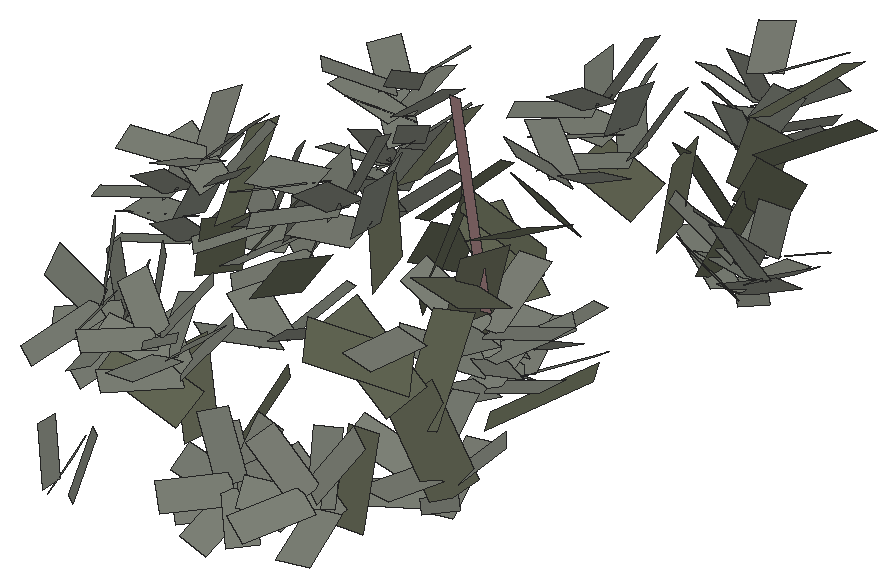
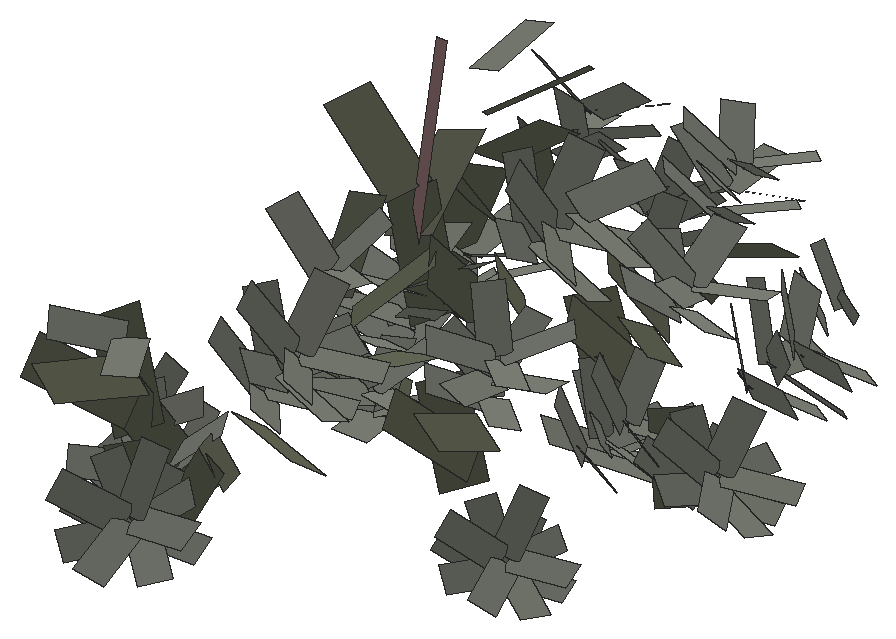
# SketchUp Ruby script. Lengths in inches.
U = 1.inch
M = Sketchup.active_model
def pt(a) = Geom::Point3d.new(a.map { |v| v * U })
def face(e, loops, mat)
  f = e.add_face(loops[0].map { |a| pt(a) })
  loops[1..].each { |l| e.add_face(l.map { |a| pt(a) }).erase! }
  f.material = f.back_material = mat if mat
  f
end
# faces: each face lists its corners as indices into pts; further lists are holes
def faces(e, pts, list, mat = nil) = list.each { |f| face(e, (f[0].is_a?(Array) ? f : [f]).map { |l| l.map { |i| pts[i] } }, mat) }
# xy, xz, yz: faces in a plane at the given z, y or x. An outline is a flat list of corners, or four numbers for a rectangle; further outlines are holes
def ring(l) = l.size == 4 ? [[l[0], l[1]], [l[2], l[1]], [l[2], l[3]], [l[0], l[3]]] : l.each_slice(2).to_a
def flat(e, list, mat, &to3) = list.each { |f| face(e, (f[0].is_a?(Array) ? f : [f]).map { |l| ring(l).map { |u, v| to3.(u, v) } }, mat) }
def xy(e, z, list, mat = nil) = flat(e, list, mat) { |x, y| [x, y, z] }
def xz(e, y, list, mat = nil) = flat(e, list, mat) { |x, z| [x, y, z] }
def yz(e, x, list, mat = nil) = flat(e, list, mat) { |y, z| [x, y, z] }
def lines(e, pts, list) = list.each { |a, b| e.add_line(pt(pts[a]), pt(pts[b])) }
# prism: a flat outline (further loops are holes) pulled along v
def prism(e, loops, v, mat = nil)
  f = face(e, loops, mat); d = Geom::Vector3d.new(v.map { |x| x * U })
  f.pushpull(f.normal.samedirection?(d) ? d.length : -d.length)
end
def box(e, o, s, mat = nil) = prism(e, [[o, [o[0] + s[0], o[1], o[2]], [o[0] + s[0], o[1] + s[1], o[2]], [o[0], o[1] + s[1], o[2]]]], [0, 0, s[2]], mat)
def at(x, y, z, deg = 0) = Geom::Transformation.translation(pt([x, y, z])) * Geom::Transformation.rotation(ORIGIN, Z_AXIS, deg.degrees)
def axes(o, x, y, z) = Geom::Transformation.new([*x, 0, *y, 0, *z, 0, *pt(o).to_a, 1])
def part(name) = M.definitions.add(name)
# library, detail: a bought-in or finely detailed component or shape, given as its bounding box
def library(name, o, s) = part(name).tap { |d| box(d.entities, o, s) }
def detail(e, o, s) = box(e.add_group.entities, o, s)
def put(e, d, t, mat = nil) = e.add_instance(d, t).tap { |i| i.material = mat if mat }
def group(e, t, mat = nil) = e.add_group.tap { |g| g.transformation = t; g.material = mat if mat }.entities
root = M.entities
M.materials.add("tak1dsfasd0f156w").color = [150, 118, 119]
M.materials.add("viburnumblaasdfas0df1w06d").color = [98, 102, 84]
M.materials.add("viburnumbladsadfasdfad0w122").color = [125, 129, 119]
c1 = part("Component\#315")
p = [[0.25,0,0],[2.05,0.01,0.35],[1.81,4.2,1.66],[0,4.19,1.3125]]
faces(c1.entities,p,[[0,1,2,3]],"viburnumbladsadfasdfad0w122")
c2 = part("viburnumblad2")
put(c2.entities,c1,axes([-19.23,-4.49,-32.18],[83.35428,0,0],[0,79.38502,0],[0,0,83.35428]))
c3 = part("Component\#314")
p = [[0.14,0,0],[2.58,0.05,0.25],[2.44,5.11,2.64],[0,5.05,2.39]]
faces(c3.entities,p,[[0,1,2,3]],"viburnumblaasdfas0df1w06d")
c4 = part("viburnumblad1\#2")
put(c4.entities,c3,axes([-37.25,6.23,19.31],[75.98784,0,0],[0,65.50676,0],[0,0,75.98784]))
c5 = part("Component\#337")
p = [[0.6,0,12.07],[1.51,1.22,0.03],[0.91,1.23,0],[0,0,12.04]]
faces(c5.entities,p,[[0,1,2,3]],"tak1dsfasd0f156w")
put(root,c2,axes([1233.48,184.79,34.33],[-0.00995,0.00489,0.00397],[-0.00628,-0.00876,-0.0047],[0.00102,-0.00608,0.00892]))
put(root,c2,axes([1233.86,186.39,33.78],[-0.01153,-0.00217,-0.00126],[0.00257,-0.00998,-0.00587],[-0.00007,-0.00594,0.00905]))
put(root,c2,axes([1227.22,186.21,31.97],[-0.00593,0.00534,0.00783],[-0.0086,-0.00691,-0.00181],[0.00397,-0.00698,0.00778]))
put(root,c2,axes([1232.86,185.47,33.13],[-0.00254,0.00908,0.00688],[-0.01141,-0.00302,-0.00024],[0.00165,-0.00679,0.00837]))
put(root,c2,axes([1227.72,187.22,32.82],[-0.00902,-0.00601,-0.00274],[0.00624,-0.00625,-0.00686],[0.00215,-0.00706,0.0084]))
put(root,c2,axes([1231.99,184.72,34.32],[0.00636,0.00796,0.00575],[-0.00984,0.00398,0.00495],[0.00146,-0.00765,0.00773]))
put(root,c2,axes([1215.61,186.57,29.77],[0.00345,-0.00905,-0.004],[0.00788,-0.00012,0.00668],[-0.00594,-0.00519,0.00581]))
put(root,c2,axes([1227.25,187.8,31.45],[-0.01058,-0.00047,0.0036],[-0.00191,-0.00936,-0.00683],[0.00314,-0.00674,0.00835]))
put(root,c2,axes([1231.93,185.9,35.2],[0.00995,-0.00489,-0.00397],[0.00634,0.00703,0.00672],[-0.00053,-0.00802,0.00751]))
put(root,c2,axes([1214.98,185.86,28.87],[0.00855,0.00051,0.00592],[-0.00403,0.00835,0.00477],[-0.00448,-0.00623,0.00604]))
put(root,c2,axes([1226.24,187.05,31.04],[0.00218,0.00802,0.00747],[-0.00931,-0.0013,0.00412],[0.00416,-0.00766,0.007]))
put(root,c2,axes([1225.95,186.33,32.57],[0.00902,0.00601,0.00274],[-0.00554,0.00435,0.00868],[0.0036,-0.00837,0.00649]))
put(root,c2,axes([1226.29,188.11,30.18],[-0.0062,0.00558,0.00817],[-0.00774,-0.00622,-0.00163],[0.00397,-0.00698,0.00778]))
put(root,c2,axes([1215.79,186.9,28.39],[0.00848,-0.00604,0.00136],[0.00312,0.00638,0.00815],[-0.00533,-0.00595,0.00568]))
put(root,c2,axes([1231.8,186.11,33.61],[0.01153,0.00217,0.00126],[-0.00261,0.00855,0.00823],[0.00055,-0.00816,0.00738]))
put(root,c2,axes([1232.29,186.56,32.28],[0.00611,0.00764,0.00552],[-0.01063,0.0043,0.00535],[0.00146,-0.00765,0.00773]))
put(root,c2,axes([1226.45,187.34,33.43],[0.00593,-0.00534,-0.00783],[0.00931,0.00502,0.00364],[0.00177,-0.00845,0.00711]))
put(root,c2,axes([1226.68,188.44,32.37],[-0.00218,-0.00802,-0.00747],[0.01085,-0.00048,-0.00266],[0.00158,-0.00777,0.00788]))
put(root,c2,axes([1220.38,188.49,37.75],[-0.00773,0.00806,0.00054],[-0.00787,-0.00734,-0.00302],[-0.00183,-0.00247,0.01075]))
put(root,c2,axes([1221.09,189.64,36.78],[-0.01083,0.00076,-0.00267],[-0.00024,-0.01097,-0.00215],[-0.00276,-0.00202,0.01064]))
put(root,c2,axes([1220.6,189.8,38.24],[-0.00759,-0.00699,-0.00431],[0.00733,-0.00841,0.00072],[-0.00369,-0.00233,0.01029]))
put(root,c2,axes([1225.42,187.78,32.17],[0.01058,0.00047,-0.0036],[0.00255,0.00709,0.00842],[0.00261,-0.00869,0.00653]))
put(root,c2,axes([1221.08,189.65,35.28],[-0.00742,0.00774,0.00052],[-0.0085,-0.00793,-0.00326],[-0.00183,-0.00247,0.01075]))
put(root,c2,axes([1225.21,188.11,30.72],[0.0079,0.00633,0.00186],[-0.00554,0.00435,0.00868],[0.00455,-0.00767,0.00675]))
put(root,c2,axes([1220.16,188.9375,36.28],[-0.0001,0.01064,0.00343],[-0.01164,0.00037,-0.00146],[-0.00143,-0.00341,0.01055]))
put(root,c4,axes([1231.6875,189.11,30.82],[0.01273,-0.00184,0.00122],[0.00029,0.0105,0.01027],[-0.0024,-0.00896,0.00784]))
put(root,c2,axes([1220.25,190.8,36.92],[0.0001,-0.01064,-0.00343],[0.01052,-0.00118,0.00394],[-0.00407,-0.00322,0.0099]))
put(root,c2,axes([1219.03,188.81,37.5],[0.00759,0.00699,0.00431],[-0.00801,0.0076,0.00179],[-0.00181,-0.0043,0.01016]))
put(root,c2,axes([1219.25,190.12,37.98],[0.00773,-0.00806,-0.00054],[0.0072,0.00653,0.00553],[-0.00368,-0.00417,0.0097]))
put(root,c4,axes([1220.77,190.28,32.375],[0.0023,0.0101,0.00657],[-0.0138,0.00343,-0.00044],[-0.0019,-0.0063,0.01035]))
put(root,c2,axes([1219.1875,189.82,36.29],[0.01083,-0.00076,0.00267],[-0.0004,0.00932,0.00428],[-0.00274,-0.00461,0.00981]))
put(root,c2,axes([1233.8,193.38,40.56],[-0.01204,0.00026,0.00058],[-0.00039,-0.0134,-0.00212],[0.00055,-0.00198,0.01239]))
put(root,c2,axes([1219.7,189.85,35.01],[0.00793,0.00729,0.0045],[-0.00721,0.00684,0.00161],[-0.00181,-0.0043,0.01016]))
put(root,c2,axes([1219.8125,190.96,35.5],[0.00743,-0.00696,-0.00145],[0.0072,0.00653,0.00553],[-0.00282,-0.00502,0.00959]))
put(root,c4,axes([1233.05,193.24,37.29],[-0.00623,0.01061,0.0062],[-0.01365,-0.00831,0.0005],[0.00356,-0.0051,0.0123]))
put(root,c4,axes([1220.29,191.55,30.54],[0.01004,0.00303,0.00636],[-0.00636,0.01197,0.00433],[-0.00443,-0.0059,0.0098]))
put(root,c2,axes([1232.98,195.73,31.45],[-0.01249,0.00076,-0.00112],[-0.00058,-0.01239,-0.00197],[-0.00123,-0.0019,0.01236]))
put(root,c4,axes([1221.05,193.57,28.89],[0.00884,-0.00966,0.00214],[0.00883,0.00982,0.0079],[-0.00632,-0.00331,0.01118]))
put(root,c2,axes([1211.15,196.41,34.3],[-0.00449,-0.0055,-0.01006],[0.00843,-0.00922,0.00132],[-0.00807,-0.00651,0.00641]))
put(root,c4,axes([1231.65,193.61,35.17],[0.00552,0.01118,0.00587],[-0.01458,0.00491,0.00435],[0.00124,-0.00686,0.01189]))
put(root,c2,axes([1211.37,195.23,33.3],[-0.00935,0.00836,-0.00053],[-0.00531,-0.00639,-0.00919],[-0.00638,-0.00686,0.0077]))
put(root,c2,axes([1232.68,195.72,29.72],[-0.00853,0.00907,0.00165],[-0.00968,-0.00877,-0.00184],[-0.00017,-0.0024,0.01233]))
put(root,c2,axes([1232.84,197.0625,30.15],[-0.00913,-0.008,-0.00324],[0.00831,-0.00942,-0.00017],[-0.00232,-0.00227,0.01214]))
put(root,c2,axes([1212.33,196.82,33.19],[-0.00979,0.00202,-0.00749],[0.00256,-0.01065,-0.00589],[-0.00735,-0.00634,0.0073]))
put(root,c2,axes([1231.66,194.93,31.08],[0.00042,0.01207,0.00346],[-0.01255,0.00034,0.00035],[0.00024,-0.00347,0.01207]))
put(root,c4,axes([1232.73,195.87,29.4],[0.00411,0.01355,0.00465],[-0.01078,-0.00135,0.01345],[0.01091,-0.00609,0.00813]))
put(root,c2,axes([1211.24,197.99,33.31],[0.00344,-0.0098,-0.00674],[0.00895,-0.00296,0.00831],[-0.00812,-0.00729,0.00557]))
put(root,c2,axes([1213.02,197.43,31.88],[-0.00898,0.00802,-0.00051],[-0.00573,-0.0069,-0.00993],[-0.00638,-0.00686,0.0077]))
put(root,c2,axes([1209.86,196.87,33.51],[0.00935,-0.00836,0.00053],[0.0036,0.00454,0.01078],[-0.00748,-0.0082,0.00525]))
put(root,c2,axes([1211.75,196.29,32.04],[-0.00344,0.0098,0.00674],[-0.01109,0.00113,-0.00697],[-0.00574,-0.00778,0.00739]))
put(root,c2,axes([1210.08,195.69,32.51],[0.00449,0.0055,0.01006],[-0.01013,0.00737,0.00027],[-0.00579,-0.00855,0.00654]))
put(root,c2,axes([1231.21,195.7,29.54],[0.00913,0.008,0.00324],[-0.00792,0.00789,0.00285],[-0.00024,-0.00448,0.01173]))
put(root,c4,axes([1230.63,195.59,33.07],[0.0147,-0.00029,0.00242],[-0.00086,0.01575,0.00709],[-0.00232,-0.00615,0.01338]))
put(root,c2,axes([1231.27,197.39,30.07],[0.00853,-0.00907,-0.00165],[0.009,0.0076,0.00473],[-0.00239,-0.00435,0.01154]))
put(root,c2,axes([1230.79,196.23,31.36],[0.01249,-0.00076,0.00112],[0.00026,0.01157,0.0049],[-0.00133,-0.00485,0.01151]))
put(root,c2,axes([1210.62,197.23,31.875],[0.00979,-0.00202,0.00749],[-0.00391,0.00808,0.00687],[-0.00651,-0.00873,0.00566]))
put(root,c2,axes([1230.99,196.98,28.45],[0.01156,-0.00022,-0.00012],[0.00026,0.01157,0.0049],[0.00003,-0.0049,0.01157]))
put(root,c2,axes([1211.43,198.73,31.89],[0.0093,-0.00683,-0.00004],[0.0036,0.00454,0.01078],[-0.00642,-0.00906,0.00528]))
put(root,c2,axes([1211.72,197.77,31.02],[0.00469,0.00575,0.0105],[-0.00912,0.00663,0.00024],[-0.00579,-0.00855,0.00654]))
put(root,c2,axes([1220.53,202.03,41.66],[-0.00996,0.00362,-0.00815],[-0.00316,-0.01285,-0.00186],[-0.00834,0.00054,0.01043]))
put(root,c2,axes([1213.25,202.88,39.86],[-0.01164,-0.00234,-0.00409],[0.00216,-0.01246,0.00098],[-0.00402,0.00034,0.01124]))
put(root,c2,axes([1221.69,203.24,40.53],[-0.00854,-0.00651,-0.00796],[0.00449,-0.01178,0.00482],[-0.00927,0.0004,0.00962]))
put(root,c4,axes([1230.1,204.41,36.25],[-0.0155,-0.00126,0.00308],[0.00163,-0.01831,0.00072],[0.00301,0.00088,0.01554]))
put(root,c2,axes([1221.23,201.68,39.98],[-0.00554,0.01163,-0.00356],[-0.00953,-0.00658,-0.00667],[-0.00756,-0.00023,0.01102]))
put(root,c2,axes([1213.1875,203.81,38.52],[-0.00535,-0.00943,-0.00399],[0.00955,-0.00712,0.00396],[-0.00559,-0.00141,0.01047]))
put(root,c2,axes([1212.24,201.7,39.42],[-0.00261,0.01228,0.0004],[-0.01201,-0.00247,-0.00269],[-0.00228,-0.00087,0.01169]))
put(root,c2,axes([1229.85,204.45,34.3],[-0.01323,-0.00019,0.0019],[0.00023,-0.01336,0.00026],[0.00189,0.00029,0.01323]))
put(root,c2,axes([1216.49,203.57,29.84],[-0.01008,0.00703,-0.00261],[-0.00714,-0.01028,-0.00011],[-0.00193,0.00159,0.01172]))
put(root,c2,axes([1222.06,204,38.94],[-0.00096,-0.01167,-0.00375],[0.00883,-0.00372,0.00932],[-0.00998,-0.00196,0.00867]))
put(root,c2,axes([1229.51,204.84,31.14],[-0.01229,-0.00021,0.00042],[0.00023,-0.01336,0.00026],[0.00045,0.00027,0.01335]))
put(root,c2,axes([1229.3125,203.79,32.59],[-0.00935,0.00927,0.0023],[-0.00914,-0.00973,0.00201],[0.00303,-0.00016,0.01302]))
put(root,c2,axes([1219.34,201.47,40.59],[0.00212,0.01282,0.00311],[-0.01094,0.00347,-0.00685],[-0.00738,-0.00146,0.01104]))
put(root,c4,axes([1215.92,205.26,31.47],[-0.00759,-0.01277,-0.00082],[0.01374,-0.0085,0.0061],[-0.0047,0.00228,0.01321]))
put(root,c2,axes([1221.78,201.92,38.3],[0.00203,0.01231,0.00299],[-0.01181,0.00375,-0.0074],[-0.00738,-0.00146,0.01104]))
put(root,c2,axes([1211.84,203.875,39.46],[0.00261,-0.01228,-0.0004],[0.01019,0.002,0.00499],[-0.00512,-0.00144,0.01069]))
put(root,c2,axes([1216.47,205.15,29.8125],[-0.00685,-0.0104,-0.00154],[0.00967,-0.00694,0.00401],[-0.00399,0.00118,0.01121]))
put(root,c2,axes([1229.31,205.67,32.74],[-0.00935,-0.00954,0.00039],[0.00874,-0.00859,-0.00062],[0.00075,-0.0002,0.01334]))
put(root,c5,axes([1227.54,203.17,35.54],[1.0472,0,0],[0,1.0472,0],[0,0,1.0472]))
put(root,c2,axes([1220.3125,203.75,39.35],[0.00554,-0.01163,0.00356],[0.00681,0.00581,0.00839],[-0.00964,-0.00181,0.00908]))
put(root,c4,axes([1229.08,205.49,39.14],[-0.00531,-0.01357,0.00158],[0.01582,-0.00598,0.00178],[-0.00086,0.00203,0.01449]))
put(root,c2,axes([1212.16,202.15,37.875],[0.00613,0.00993,0.00305],[-0.0113,0.00738,-0.00131],[-0.00247,-0.00201,0.01151]))
put(root,c4,axes([1227.6875,205.5,32.59],[-0.00382,-0.01538,-0.00062],[0.0121,-0.00355,0.01339],[-0.01131,0.00237,0.01086]))
put(root,c2,axes([1228.49,203.46,34.4],[0,0.0133,0.00135],[-0.0129,-0.00035,0.00349],[0.0035,-0.0013,0.01283]))
put(root,c2,axes([1220.15,202.21,39.07],[0.00854,0.00651,0.00796],[-0.00689,0.01199,-0.00242],[-0.00792,-0.00244,0.01048]))
put(root,c2,axes([1211.9375,203.73,38.01],[0.01052,-0.00734,0.00272],[0.0053,0.00911,0.00408],[-0.00448,-0.00242,0.01081]))
put(root,c2,axes([1211.18,202.6,39.13],[0.01164,0.00234,0.00409],[-0.0032,0.01265,0.00186],[-0.00338,-0.00265,0.01114]))
put(root,c2,axes([1228.89,205.81,34.58],[0,-0.0133,-0.00135],[0.01336,0.00003,-0.00028],[0.00028,-0.00135,0.01329]))
put(root,c2,axes([1221.14,203.46,37.97],[0.01039,-0.00378,0.00851],[0.00094,0.01134,0.00389],[-0.00886,-0.00258,0.00967]))
put(root,c2,axes([1228.62,205.97,31.28],[0,-0.01388,-0.00141],[0.01203,0.00003,-0.00025],[0.00028,-0.00135,0.01329]))
put(root,c2,axes([1214.95,203.54,29.46],[0.00685,0.0104,0.00154],[-0.01034,0.00702,-0.00117],[-0.00153,-0.00054,0.01185]))
put(root,c4,axes([1223.2,203.09,35.24],[0.00849,0.00329,0.01149],[-0.00585,0.01597,-0.00025],[-0.01083,-0.00383,0.0091]))
put(root,c4,axes([1212.54,203.52,34.99],[0.01199,-0.00124,0.00662],[-0.00048,0.01553,0.00369],[-0.00665,-0.00299,0.01093]))
put(root,c4,axes([1213.63,204.95,33.3],[0.0067,-0.01138,0.00383],[0.01125,0.009,0.0069],[-0.00701,-0.00007,0.01111]))
put(root,c2,axes([1227.63,204.02,32.86],[0.00935,0.00954,-0.00039],[-0.00905,0.00903,0.00388],[0.00303,-0.00246,0.01278]))
put(root,c2,axes([1212.76,208.16,34.51],[-0.00608,-0.00542,-0.00802],[0.00543,-0.00975,0.00248],[-0.00802,-0.0025,0.00776]))
put(root,c2,axes([1208.39,207.9,31.62],[-0.00935,-0.0054,-0.00582],[0.00241,-0.00918,0.00416],[-0.00697,0.00288,0.00746]))
put(root,c2,axes([1214.93,205.125,29.43],[0.01008,-0.00703,0.00261],[0.00646,0.01036,0.00294],[-0.0036,-0.00095,0.01134]))
put(root,c4,axes([1224.71,204.68,33.62],[0.00719,-0.00894,0.00913],[0.00526,0.01343,0.009],[-0.01194,-0.00098,0.00844]))
put(root,c2,axes([1213.8,208.02,33.32],[-0.0088,0.00279,-0.00674],[-0.00068,-0.01083,-0.00359],[-0.00727,-0.00236,0.00851]))
put(root,c2,axes([1227.76,205.52,32.97],[0.00935,-0.00927,-0.0023],[0.00999,0.00977,0.00128],[0.00075,-0.00249,0.01311]))
put(root,c2,axes([1207.65,207.66,32.62],[-0.00882,0.00375,-0.00654],[-0.00425,-0.0099,-0.00033],[-0.00607,0.00296,0.00807]))
put(root,c2,axes([1212.6,206.91,33.79],[-0.00637,0.00937,-0.00151],[-0.00692,-0.00583,-0.00699],[-0.0065,-0.00298,0.00892]))
put(root,c2,axes([1206.83,208.52,33.6],[-0.00896,-0.00518,-0.00557],[0.00268,-0.0102,0.00462],[-0.00697,0.00288,0.00746]))
put(root,c4,axes([1209.9,208.02,29.4375],[-0.0079,-0.01009,-0.00146],[0.00852,-0.00752,0.00905],[-0.00687,0.00486,0.00819]))
put(root,c2,axes([1207.8125,206.77,31.45],[-0.00267,0.00936,-0.00422],[-0.0097,-0.00494,-0.00456],[-0.00579,0.00336,0.00814]))
put(root,c2,axes([1227.53,204.82,34.68],[0.01323,0.00019,-0.0019],[0.00023,0.01303,0.00294],[0.00189,-0.00295,0.0129]))
put(root,c2,axes([1227.33,204.86,31.3125],[0.0127,0.00018,-0.00182],[0.00025,0.01408,0.00318],[0.00189,-0.00295,0.0129]))
put(root,c4,axes([1227.47,206.33,28.06],[0.00753,-0.01256,0.00063],[0.01453,0.00876,0.0012],[-0.00121,0,0.01461]))
put(root,c2,axes([1206.16,207.22,33.29],[-0.00351,0.01047,-0.00368],[-0.0097,-0.00494,-0.00456],[-0.00545,0.00224,0.00858]))
put(root,c2,axes([1228.4375,209.36,29.64],[-0.01209,-0.0034,-0.0003],[0.00332,-0.01209,0.00349],[-0.00129,0.00365,0.01095]))
put(root,c2,axes([1228.27,208.72,31.22],[-0.01088,0.00599,-0.0016],[-0.00628,-0.01045,0.00254],[-0.00013,0.00352,0.01104]))
put(root,c2,axes([1207.14,208.84,32.14],[-0.00385,-0.01107,-0.00134],[0.00835,-0.0037,0.00784],[-0.00761,0.00206,0.00711]))
put(root,c2,axes([1214.43,208.15,31.93],[-0.00611,0.009,-0.00145],[-0.00747,-0.0063,-0.00755],[-0.0065,-0.00298,0.00892]))
put(root,c2,axes([1213.11,209.32,33.28],[0.00021,-0.01046,-0.0046],[0.00792,-0.00325,0.00774],[-0.00831,-0.0033,0.00712]))
put(root,c2,axes([1206.36,206.9375,31.85],[0.00385,0.01107,0.00134],[-0.00965,0.00395,-0.00558],[-0.00546,0.00115,0.0087]))
put(root,c2,axes([1213.07,207.51,32.39],[-0.00021,0.01046,0.0046],[-0.01011,0.00244,-0.006],[-0.00617,-0.00398,0.00877]))
put(root,c2,axes([1227.81,208.04,29.78],[-0.0033,0.01188,-0.00196],[-0.01112,-0.00285,0.00099],[0.00058,0.00262,0.01122]))
put(root,c2,axes([1228.12,210.27,30.99],[-0.00622,-0.0108,0.00117],[0.01069,-0.00568,0.00296],[-0.00222,0.00293,0.01099]))
put(root,c2,axes([1211.66,208.73,33.77],[0.00637,-0.00937,0.00151],[0.00514,0.00494,0.00894],[-0.00798,-0.0043,0.00697]))
put(root,c2,axes([1207.34,208.48,30.78],[0.00337,-0.01006,0.00353],[0.00874,0.00576,0.00702],[-0.00763,0.00098,0.00722]))
put(root,c2,axes([1211.5,207.49,33.05],[0.00608,0.00542,0.00802],[-0.00721,0.00886,-0.00053],[-0.00646,-0.00478,0.00813]))
put(root,c4,axes([1228.3,209.79,35.03],[-0.00837,0.01093,-0.00027],[-0.01213,-0.00903,0.00454],[0.00324,0.00308,0.01192]))
put(root,c2,axes([1205.82,209.23,32.82],[0.00351,-0.01047,0.00368],[0.00809,0.00534,0.0065],[-0.00763,0.00098,0.00722]))
put(root,c2,axes([1212.28,208.57,32.125],[0.0088,-0.00279,0.00674],[-0.001,0.00912,0.00509],[-0.00721,-0.00491,0.00738]))
put(root,c2,axes([1213.32,209.66,31.8],[0.00662,-0.00815,0.00069],[0.00514,0.00494,0.00894],[-0.00725,-0.00529,0.00709]))
put(root,c4,axes([1228.71,211.65,36.625],[-0.0135,0.00082,0.00242],[0.00046,-0.01443,0.00598],[0.00274,0.00585,0.01119]))
put(root,c2,axes([1206.09,208.36,31.5],[0.00882,-0.00375,0.00654],[0.00302,0.01118,0.0023],[-0.00701,0.00026,0.00774]))
put(root,c2,axes([1205.15,207.93,32.51],[0.00896,0.00518,0.00557],[-0.00429,0.01059,-0.00268],[-0.00611,0.00033,0.00835]))
put(root,c2,axes([1227.27,210.15,29.47],[0.0033,-0.01188,0.00196],[0.01189,0.00365,0.00167],[-0.00236,0.00179,0.01115]))
put(root,c2,axes([1213.29,208.6,31.15],[0.00634,0.00566,0.00838],[-0.00649,0.00797,-0.00047],[-0.00646,-0.00478,0.00813]))
put(root,c2,axes([1226.69,208.55,31.14],[0.00622,0.0108,-0.00117],[-0.01091,0.00622,-0.00021],[0.00044,0.00147,0.01138]))
put(root,c4,axes([1226.71,208.84,32.81],[0.00652,0.01335,-0.00071],[-0.01553,0.00758,0.00028],[0.00058,0.00086,0.01356]))
put(root,c2,axes([1226.27,208.89,29.58],[0.01209,0.0034,0.0003],[-0.00342,0.01218,-0.00058],[-0.00049,0.00075,0.01143]))
put(root,c2,axes([1228.375,212.08,39.54],[-0.01136,0.00626,-0.00167],[-0.00561,-0.00886,0.00368],[0.00077,0.00497,0.01057]))
put(root,c2,axes([1226.54,210.11,30.91],[0.01088,-0.00599,0.0016],[0.00606,0.01099,0.00021],[-0.00165,0.00089,0.01133]))
put(root,c2,axes([1228.09,213.57,39.1],[-0.00603,-0.00996,0.00266],[0.01166,-0.00593,0.00316],[-0.00133,0.00444,0.01071]))
put(root,c4,axes([1218.73,214.1,29.85],[-0.00965,-0.00928,0.0022],[0.01068,-0.00958,0.00645],[-0.00246,0.00545,0.01217]))
put(root,c2,axes([1216.57,214.2,38.31],[-0.01113,0.0001,-0.00261],[-0.00085,-0.01106,0.00319],[-0.00248,0.00327,0.01067]))
put(root,c2,axes([1216.61,214.77,36.88],[-0.0072,-0.00751,-0.00155],[0.00713,-0.00775,0.00446],[-0.00433,0.00201,0.01039]))
put(root,c2,axes([1215.66,213.72,39.69],[-0.00749,0.00804,-0.00315],[-0.0085,-0.00761,0.00079],[-0.00154,0.00286,0.01096]))
put(root,c2,axes([1215.96,215.12,39.52],[-0.00825,-0.0079,-0.00055],[0.00713,-0.00775,0.00446],[-0.00345,0.00288,0.01051]))
put(root,c2,axes([1227.03,211.93,39.67],[0.00561,0.0092,-0.00364],[-0.0108,0.0064,-0.00025],[0.002,0.00408,0.01074]))
put(root,c2,axes([1215.38,213.35,38.18],[0.00053,0.01127,-0.00184],[-0.01136,0.00033,-0.00126],[-0.00119,0.00188,0.01121]))
put(root,c2,axes([1215.52,215.33,37.83],[-0.00053,-0.01127,0.00184],[0.00985,0.00012,0.00361],[-0.0039,0.00191,0.01058]))
put(root,c2,axes([1215.27,213.48,36.66],[0.00792,0.00758,0.00053],[-0.00837,0.00887,-0.00193],[-0.00163,0.00092,0.01128]))
put(root,c2,axes([1215.45,214.92,36.49],[0.00782,-0.00839,0.00329],[0.00709,0.00727,0.00169],[-0.00355,0.00093,0.01083]))
put(root,c4,axes([1216.8,214.72,31.76],[0.00364,-0.01074,0.00535],[0.01254,0.00622,0.00396],[-0.00521,0.00362,0.01082]))
put(root,c2,axes([1214.28,213.98,39.33],[0.00825,0.0079,0.00055],[-0.00775,0.00821,-0.00179],[-0.00163,0.00092,0.01128]))
put(root,c2,axes([1214.59,215.375,39.16],[0.00749,-0.00804,0.00315],[0.00787,0.00807,0.00188],[-0.00355,0.00093,0.01083]))
put(root,c2,axes([1214.62,214.33,37.81],[0.01113,-0.0001,0.00261],[0.00023,0.01199,-0.00051],[-0.00261,0.00052,0.01112]))
put(root,c4,axes([1215.66,214.06,33.6875],[0.01084,-0.00282,0.00565],[0.00343,0.01413,0.00046],[-0.00557,0.00099,0.01119]))
put(root,c2,axes([1212.72,218.23,29.96],[-0.00996,-0.0034,-0.00378],[0.0004,-0.00774,0.0055],[-0.00482,0.0055,0.00684]))
put(root,c2,axes([1212.1,218.39,30.98],[-0.00747,0.00421,-0.00626],[-0.00602,-0.00754,0.00188],[-0.00396,0.00545,0.00734]))
put(root,c2,axes([1211.94,217.38,30.06],[-0.00059,0.00795,-0.00557],[-0.01005,-0.00269,-0.00267],[-0.00362,0.00574,0.0073]))
put(root,c2,axes([1225.36,219.56,38.29],[-0.00962,0.00434,-0.00682],[-0.00417,-0.01174,-0.00159],[-0.00692,0.00104,0.01043]))
put(root,c2,axes([1224.49,220.19,39.65],[-0.00913,-0.00526,-0.00683],[0.00354,-0.01136,0.00402],[-0.00787,0.001,0.00974]))
put(root,c2,axes([1211.66,219.51,31.79],[-0.00954,-0.00326,-0.00362],[0.00044,-0.00861,0.00611],[-0.00482,0.0055,0.00684]))
put(root,c2,axes([1211.88,219.45,30.34],[-0.00602,-0.00882,0.00114],[0.00718,-0.00382,0.00749],[-0.0056,0.00489,0.00671]))
put(root,c2,axes([1223.87,218.82,39.15],[-0.00447,0.0114,-0.0028],[-0.00996,-0.00527,-0.00554],[-0.00621,0.00025,0.01092]))
put(root,c2,axes([1210.75,218.5,31.79],[-0.00103,0.00921,-0.00523],[-0.01005,-0.00269,-0.00267],[-0.00353,0.00478,0.00792]))
put(root,c2,axes([1211.85,218.85,29.125],[0.00099,-0.00884,0.00502],[0.00961,0.00407,0.00487],[-0.00586,0.00398,0.00703]))
put(root,c2,axes([1225.83,219.28,36.7],[-0.00429,0.01094,-0.00269],[-0.01076,-0.0057,-0.00599],[-0.00621,0.00025,0.01092]))
put(root,c2,axes([1210.74,217.94,30.49],[0.00602,0.00882,-0.00114],[-0.00807,0.00476,-0.00535],[-0.00378,0.00387,0.00824]))
put(root,c2,axes([1224.97,221.1,38.06],[-0.0033,-0.01178,-0.00285],[0.00874,-0.0044,0.00808],[-0.00849,0.00014,0.00926]))
put(root,c2,axes([1233.92,220.99,32.27],[-0.01012,-0.0002,-0.00445],[-0.00314,-0.00766,0.00749],[-0.00319,0.00804,0.00689]))
put(root,c2,axes([1210.86,220.22,30.98],[0.00103,-0.00921,0.00523],[0.0089,0.00377,0.00451],[-0.00586,0.00398,0.00703]))
put(root,c2,axes([1231.54,221.6,30.07],[-0.01209,0.00339,-0.00041],[-0.00309,-0.0102,0.00689],[0.00151,0.00666,0.01054]))
put(root,c2,axes([1210.79,219.18,29.9],[0.00747,-0.00421,0.00626],[0.0054,0.00929,-0.00022],[-0.00543,0.00331,0.00761]))
put(root,c2,axes([1224.3,219.07,37.47],[0.0033,0.01178,0.00285],[-0.01097,0.00447,-0.0058],[-0.00615,-0.00092,0.01092]))
put(root,c2,axes([1223.36,220.98,38.87],[0.00447,-0.0114,0.0028],[0.00817,0.00518,0.00802],[-0.00843,-0.00103,0.00925]))
put(root,c2,axes([1209.95,219.21,30.99],[0.00954,0.00326,0.00362],[-0.0016,0.00968,-0.00428],[-0.00457,0.00326,0.00811]))
put(root,c2,axes([1232.8,221.33,33.46],[-0.00525,0.00588,-0.00776],[-0.00943,-0.00525,0.0024],[-0.00241,0.00775,0.0075]))
put(root,c4,axes([1226.68,219.46,33.46],[0.00447,0.01094,0.00709],[-0.01215,0.00867,-0.00572],[-0.00776,-0.00379,0.01074]))
put(root,c2,axes([1225.04,221.15,36.375],[0.00493,-0.01032,0.00165],[0.00817,0.00518,0.00802],[-0.0079,-0.00226,0.0095]))
put(root,c2,axes([1232.67,220.33,32.3125],[0.0027,0.00851,-0.00652],[-0.01047,0.00066,-0.00347],[-0.00228,0.00703,0.00822]))
put(root,c2,axes([1231.54,223.03,31.17],[-0.01083,-0.00527,0.00359],[0.00636,-0.00933,0.00551],[0.00035,0.00657,0.01071]))
put(root,c2,axes([1233.35,222.39,32.74],[-0.00906,-0.00616,0.00146],[0.00477,-0.00497,0.00864],[-0.00416,0.00772,0.00674]))
put(root,c2,axes([1232.8,219.72,30.97],[0.0087,0.00591,-0.0014],[-0.00609,0.00723,-0.0073],[-0.00288,0.00629,0.00863]))
put(root,c2,axes([1222.74,219.61,38.36],[0.00913,0.00526,0.00683],[-0.00534,0.01127,-0.00154],[-0.00678,-0.00178,0.01043]))
put(root,c2,axes([1223.7,220.36,37.07],[0.00962,-0.00434,0.00682],[0.00218,0.01069,0.00373],[-0.00772,-0.00183,0.00974]))
put(root,c2,axes([1224.62,219.95,35.9],[0.00954,0.0055,0.00713],[-0.0048,0.01014,-0.00139],[-0.00678,-0.00178,0.01043]))
put(root,c2,axes([1230.88,221.75,31.84],[-0.00627,0.01006,-0.00416],[-0.01061,-0.00457,0.00494],[0.00244,0.00598,0.01078]))
put(root,c2,axes([1230.66,223,29.45],[-0.00322,-0.01084,0.00548],[0.01114,-0.00248,0.00163],[-0.00036,0.00575,0.01116]))
put(root,c4,axes([1231.6,223.92,32.78],[-0.01228,-0.00656,0.00533],[0.00976,-0.01204,0.00766],[0.00081,0.00845,0.01225]))
put(root,c2,axes([1230.05,221.125,30.45],[0.00322,0.01084,-0.00548],[-0.01186,0.00402,0.00097],[0.00259,0.00493,0.01126]))
put(root,c2,axes([1232.18,221.03,31.41],[0.01012,0.0002,0.00445],[0.00236,0.00977,-0.0058],[-0.00385,0.00596,0.00848]))
put(root,c4,axes([1229.43,222.09,29.63],[0.00407,-0.01295,0.00616],[0.01043,0.00846,0.01089],[-0.01117,0.00115,0.0098]))
put(root,c4,axes([1227.31,220.6,31.25],[0.00927,0.00064,0.01018],[-0.00266,0.0157,0.00144],[-0.00994,-0.00253,0.00921]))
put(root,c2,axes([1231.6,221.49,32.76],[0.00906,0.00616,-0.00146],[-0.00564,0.00669,-0.00676],[-0.00288,0.00629,0.00863]))
put(root,c2,axes([1230.11,223.68,31],[0.00627,-0.01006,0.00416],[0.01088,0.00589,-0.00218],[-0.0002,0.0047,0.01165]))
put(root,c2,axes([1229.44,222.3,29.92],[0.01209,-0.00339,0.00041],[0.0035,0.01198,-0.00427],[0.00073,0.00402,0.01188]))
put(root,c2,axes([1229.44,222.41,31.67],[0.01083,0.00527,-0.00359],[-0.00609,0.01064,-0.00276],[0.00188,0.00411,0.01172]))
put(root,c4,axes([1227.74,226.45,29.88],[-0.01186,0.00394,-0.00337],[-0.00604,-0.00999,0.00917],[0.00026,0.00862,0.00831]))
put(root,c4,axes([1230.04,225.4375,34.92],[0.00185,-0.01141,0.00751],[0.01551,0.00355,0.00158],[-0.0028,0.0071,0.01148]))
put(root,c2,axes([1229.43,226.83,40.12],[0.00655,-0.0105,0.00435],[0.00967,0.00585,-0.00045],[-0.00175,0.00381,0.01184]))
put(root,c2,axes([1228.89,225.4,40.61],[0.01044,0.00574,-0.00186],[-0.00678,0.01138,-0.00292],[0.00034,0.00331,0.01211]))
put(root,c4,axes([1228.97,225.4,37.25],[0.01159,-0.00514,0.00541],[0.00744,0.01388,-0.00276],[-0.00381,0.00452,0.01245]))
put(root,c4,axes([1227.09,228.625,30.42],[-0.01156,-0.00444,0.00366],[0.00659,-0.0076,0.0107],[-0.00137,0.01006,0.00666]))
put(root,c2,axes([1226.38,230,32.73],[-0.01201,-0.00131,-0.00224],[-0.00075,-0.00731,0.00743],[-0.00252,0.0083,0.00677]))
put(root,c2,axes([1225.35,229.34,33.1],[0.00059,0.00756,-0.00753],[-0.01174,-0.00037,-0.00119],[-0.00112,0.00828,0.00709]))
put(root,c2,axes([1225.93,230.51,33.87],[-0.00777,0.00552,-0.00673],[-0.00804,-0.00584,0.00423],[-0.00155,0.00808,0.00722]))
put(root,c2,axes([1225.88,231.57,33],[-0.0085,-0.0073,0.00369],[0.00776,-0.00483,0.008],[-0.00353,0.00786,0.00685]))
put(root,c2,axes([1225.49,230.75,31.8125],[-0.0005,-0.0087,0.00708],[0.01199,0.0023,0.00332],[-0.00399,0.00704,0.00741]))
put(root,c2,axes([1225.9,231.9375,34.56],[-0.01151,-0.00126,-0.00215],[-0.00083,-0.00812,0.00826],[-0.00252,0.0083,0.00677]))
put(root,c2,axes([1224.67,231.15,34.875],[0.00052,0.00907,-0.00737],[-0.01174,-0.00037,-0.00119],[-0.00118,0.00734,0.00793]))
put(root,c2,axes([1224.3,230.36,33.59],[0.0085,0.0073,-0.00369],[-0.00811,0.00643,-0.0058],[-0.00164,0.00652,0.00849]))
put(root,c2,axes([1224.59,231.53,32.7],[0.00777,-0.00552,0.00673],[0.00812,0.00813,-0.00272],[-0.00362,0.0063,0.00812]))
put(root,c2,axes([1225.11,232.78,33.64],[-0.00052,-0.00907,0.00737],[0.0111,0.00213,0.00308],[-0.00399,0.00704,0.00741]))
put(root,c2,axes([1223.89,231.99,33.96],[0.01151,0.00126,0.00215],[0.0002,0.00988,-0.00637],[-0.00265,0.00609,0.00857]))
